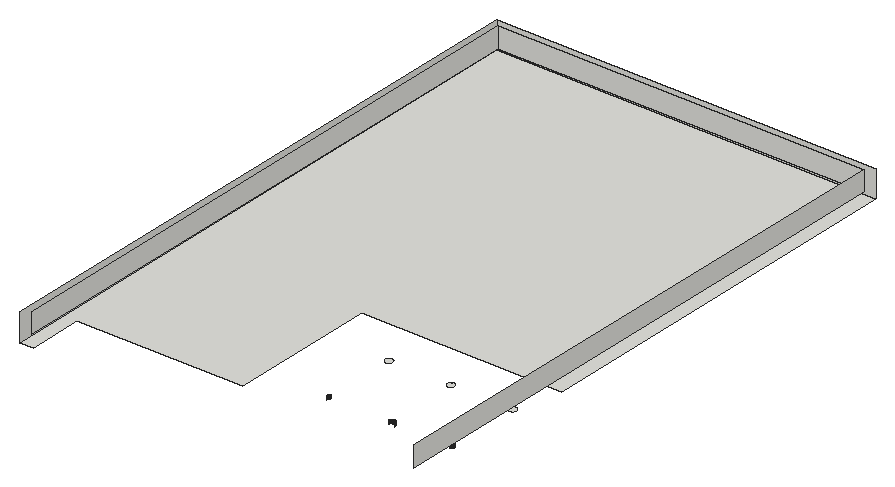
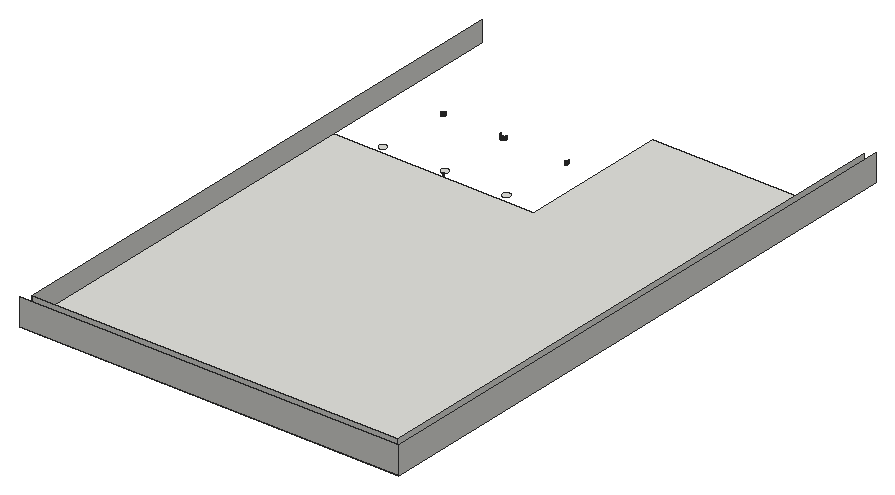
# SketchUp Ruby script. Lengths in inches.
U = 1.inch
M = Sketchup.active_model
def pt(a) = Geom::Point3d.new(a.map { |v| v * U })
def face(e, loops, mat)
  f = e.add_face(loops[0].map { |a| pt(a) })
  loops[1..].each { |l| e.add_face(l.map { |a| pt(a) }).erase! }
  f.material = f.back_material = mat if mat
  f
end
# faces: each face lists its corners as indices into pts; further lists are holes
def faces(e, pts, list, mat = nil) = list.each { |f| face(e, (f[0].is_a?(Array) ? f : [f]).map { |l| l.map { |i| pts[i] } }, mat) }
# xy, xz, yz: faces in a plane at the given z, y or x. An outline is a flat list of corners, or four numbers for a rectangle; further outlines are holes
def ring(l) = l.size == 4 ? [[l[0], l[1]], [l[2], l[1]], [l[2], l[3]], [l[0], l[3]]] : l.each_slice(2).to_a
def flat(e, list, mat, &to3) = list.each { |f| face(e, (f[0].is_a?(Array) ? f : [f]).map { |l| ring(l).map { |u, v| to3.(u, v) } }, mat) }
def xy(e, z, list, mat = nil) = flat(e, list, mat) { |x, y| [x, y, z] }
def xz(e, y, list, mat = nil) = flat(e, list, mat) { |x, z| [x, y, z] }
def yz(e, x, list, mat = nil) = flat(e, list, mat) { |y, z| [x, y, z] }
def lines(e, pts, list) = list.each { |a, b| e.add_line(pt(pts[a]), pt(pts[b])) }
# prism: a flat outline (further loops are holes) pulled along v
def prism(e, loops, v, mat = nil)
  f = face(e, loops, mat); d = Geom::Vector3d.new(v.map { |x| x * U })
  f.pushpull(f.normal.samedirection?(d) ? d.length : -d.length)
end
def box(e, o, s, mat = nil) = prism(e, [[o, [o[0] + s[0], o[1], o[2]], [o[0] + s[0], o[1] + s[1], o[2]], [o[0], o[1] + s[1], o[2]]]], [0, 0, s[2]], mat)
def at(x, y, z, deg = 0) = Geom::Transformation.translation(pt([x, y, z])) * Geom::Transformation.rotation(ORIGIN, Z_AXIS, deg.degrees)
def axes(o, x, y, z) = Geom::Transformation.new([*x, 0, *y, 0, *z, 0, *pt(o).to_a, 1])
def part(name) = M.definitions.add(name)
# library, detail: a bought-in or finely detailed component or shape, given as its bounding box
def library(name, o, s) = part(name).tap { |d| box(d.entities, o, s) }
def detail(e, o, s) = box(e.add_group.entities, o, s)
def put(e, d, t, mat = nil) = e.add_instance(d, t).tap { |i| i.material = mat if mat }
def group(e, t, mat = nil) = e.add_group.tap { |g| g.transformation = t; g.material = mat if mat }.entities
root = M.entities
xy(root,234,[[214.28,317,214.2,317.01,214.12,317.01,213.96,317.03,213.89,317.04,213.73,317.08,213.66,317.09,213.58,317.11,213.5,317.14,213.43,317.16,213.36,317.1875,213.28,317.22,213.14,317.28,213.07,317.3125,213,317.35,212.93,317.39,212.86,317.42,212.79,317.47,212.73,317.51,212.66,317.55,212.36,317.8,212.19,317.97,211.99,318.21,211.95,318.27,211.9,318.34,211.86,318.4,211.74,318.61,211.71,318.68,211.67,318.75,211.61,318.89,211.58,318.97,211.56,319.04,211.53,319.12,211.51,319.19,211.49,319.27,211.47,319.34,211.46,319.42,211.44,319.5,211.43,319.58,211.42,319.65,211.41,319.73,211.41,319.81,211.4,319.89,211.4,320.125,211.41,320.2,211.41,320.28,211.42,320.36,211.43,320.4375,211.44,320.51,211.48,320.67,211.49,320.74,211.51,320.82,211.54,320.9,211.5625,320.97,211.59,321.04,211.62,321.12,211.71,321.33,211.79,321.47,211.82,321.54,211.87,321.61,211.91,321.67,211.95,321.74,212.2,322.04,212.26,322.1,212.3125,322.15,212.37,322.21,212.61,322.41,212.67,322.45,212.74,322.5,212.8,322.54,212.87,322.58,212.9375,322.62,213.01,322.66,213.08,322.69,213.15,322.73,213.29,322.79,213.37,322.82,213.44,322.84,213.52,322.87,213.59,322.89,213.67,322.91,213.74,322.93,213.82,322.94,213.9,322.96,213.98,322.97,214.05,322.98,214.13,322.99,214.21,322.99,214.29,323,214.52,323,214.6,322.99,214.68,322.99,214.84,322.97,214.91,322.96,215.07,322.92,215.14,322.91,215.22,322.89,215.3,322.86,215.37,322.84,215.44,322.8125,215.52,322.78,215.66,322.72,215.73,322.6875,215.8,322.65,215.87,322.61,215.9375,322.58,216.01,322.53,216.07,322.49,216.14,322.45,216.44,322.2,216.61,322.03,216.81,321.79,216.85,321.73,216.9,321.66,216.94,321.6,217.06,321.39,217.09,321.32,217.16,321.18,217.1875,321.11,217.22,321.03,217.24,320.96,217.27,320.88,217.29,320.81,217.31,320.73,217.33,320.66,217.34,320.58,217.36,320.5,217.37,320.42,217.38,320.35,217.39,320.27,217.39,320.19,217.4,320.11,217.4,319.875,217.39,319.8,217.39,319.72,217.38,319.64,217.37,319.5625,217.36,319.49,217.32,319.33,217.31,319.26,217.29,319.18,217.26,319.1,217.24,319.03,217.21,318.96,217.18,318.88,217.09,318.67,217.01,318.53,216.98,318.46,216.93,318.39,216.89,318.33,216.85,318.26,216.6,317.96,216.43,317.79,216.375,317.74,216.25,317.64,216.19,317.59,216.125,317.55,216.0625,317.5,216,317.46,215.79,317.34,215.72,317.31,215.65,317.27,215.51,317.21,215.43,317.18,215.36,317.16,215.28,317.13,215.21,317.11,215.13,317.09,215.06,317.07,214.98,317.06,214.9,317.04,214.82,317.03,214.75,317.02,214.67,317.01,214.59,317.01,214.51,317],[269.08,317,269,317.01,268.92,317.01,268.76,317.03,268.6875,317.04,268.61,317.06,268.53,317.08,268.46,317.09,268.38,317.11,268.3,317.14,268.23,317.16,268.16,317.1875,268.08,317.22,268.01,317.25,267.9375,317.28,267.87,317.3125,267.8,317.35,267.73,317.39,267.66,317.42,267.59,317.47,267.53,317.51,267.46,317.55,267.16,317.8,266.99,317.97,266.79,318.21,266.75,318.27,266.7,318.34,266.66,318.4,266.54,318.61,266.51,318.68,266.47,318.75,266.41,318.89,266.38,318.97,266.36,319.04,266.33,319.12,266.3125,319.19,266.29,319.27,266.27,319.34,266.26,319.42,266.24,319.5,266.23,319.58,266.22,319.65,266.21,319.73,266.21,319.81,266.2,319.89,266.2,320.125,266.21,320.2,266.21,320.28,266.22,320.36,266.23,320.4375,266.24,320.51,266.28,320.67,266.29,320.74,266.3125,320.82,266.34,320.9,266.36,320.97,266.39,321.04,266.42,321.12,266.51,321.33,266.59,321.47,266.625,321.54,266.67,321.61,266.71,321.67,266.75,321.74,267,322.04,267.17,322.21,267.41,322.41,267.47,322.45,267.54,322.5,267.6,322.54,267.81,322.66,267.88,322.69,267.95,322.73,268.09,322.79,268.17,322.82,268.24,322.84,268.32,322.87,268.39,322.89,268.47,322.91,268.54,322.93,268.62,322.94,268.7,322.96,268.78,322.97,268.85,322.98,268.93,322.99,269.01,322.99,269.09,323,269.32,323,269.4,322.99,269.48,322.99,269.64,322.97,269.71,322.96,269.87,322.92,269.94,322.91,270.02,322.89,270.1,322.86,270.17,322.84,270.24,322.8125,270.32,322.78,270.46,322.72,270.53,322.6875,270.6,322.65,270.67,322.61,270.74,322.58,270.81,322.53,270.87,322.49,270.9375,322.45,271.0625,322.35,271.12,322.3,271.24,322.2,271.41,322.03,271.61,321.79,271.65,321.73,271.7,321.66,271.74,321.6,271.86,321.39,271.89,321.32,271.93,321.25,271.99,321.11,272.02,321.03,272.04,320.96,272.07,320.88,272.09,320.81,272.11,320.73,272.13,320.66,272.14,320.58,272.16,320.5,272.17,320.42,272.18,320.35,272.1875,320.27,272.19,320.19,272.2,320.11,272.2,319.875,272.19,319.8,272.1875,319.72,272.18,319.64,272.17,319.5625,272.16,319.49,272.14,319.41,272.125,319.33,272.11,319.26,272.09,319.18,272.0625,319.1,272.04,319.03,272.01,318.96,271.98,318.88,271.89,318.67,271.81,318.53,271.78,318.46,271.73,318.39,271.69,318.33,271.65,318.26,271.4,317.96,271.23,317.79,270.99,317.59,270.93,317.55,270.86,317.5,270.8,317.46,270.59,317.34,270.52,317.31,270.45,317.27,270.31,317.21,270.23,317.18,270.16,317.16,270.08,317.13,270.01,317.11,269.93,317.09,269.86,317.07,269.78,317.06,269.7,317.04,269.55,317.02,269.47,317.01,269.39,317.01,269.3125,317],[323.875,317,323.8,317.01,323.72,317.01,323.64,317.02,323.5625,317.03,323.49,317.04,323.33,317.08,323.26,317.09,323.18,317.11,323.1,317.14,323.03,317.16,322.96,317.1875,322.88,317.22,322.74,317.28,322.67,317.3125,322.6,317.35,322.53,317.39,322.46,317.42,322.39,317.47,322.33,317.51,322.26,317.55,321.96,317.8,321.79,317.97,321.59,318.21,321.55,318.27,321.5,318.34,321.46,318.4,321.34,318.61,321.31,318.68,321.27,318.75,321.21,318.89,321.18,318.97,321.16,319.04,321.13,319.12,321.11,319.19,321.09,319.27,321.07,319.34,321.06,319.42,321.04,319.5,321.03,319.58,321.02,319.65,321.01,319.73,321.01,319.81,321,319.89,321,320.125,321.01,320.2,321.01,320.28,321.02,320.36,321.03,320.4375,321.04,320.51,321.08,320.67,321.09,320.74,321.11,320.82,321.14,320.9,321.16,320.97,321.1875,321.04,321.22,321.12,321.28,321.26,321.3125,321.33,321.35,321.4,321.39,321.47,321.42,321.54,321.47,321.61,321.51,321.67,321.55,321.74,321.8,322.04,321.97,322.21,322.21,322.41,322.27,322.45,322.34,322.5,322.4,322.54,322.61,322.66,322.68,322.69,322.75,322.73,322.89,322.79,322.97,322.82,323.04,322.84,323.12,322.87,323.19,322.89,323.27,322.91,323.34,322.93,323.42,322.94,323.5,322.96,323.58,322.97,323.65,322.98,323.73,322.99,323.81,322.99,323.89,323,324.125,323,324.2,322.99,324.28,322.99,324.36,322.98,324.4375,322.97,324.51,322.96,324.67,322.92,324.74,322.91,324.82,322.89,324.9,322.86,324.97,322.84,325.04,322.8125,325.12,322.78,325.26,322.72,325.33,322.6875,325.4,322.65,325.47,322.61,325.54,322.58,325.61,322.53,325.67,322.49,325.74,322.45,326.04,322.2,326.21,322.03,326.41,321.79,326.45,321.73,326.5,321.66,326.54,321.6,326.66,321.39,326.69,321.32,326.73,321.25,326.79,321.11,326.82,321.03,326.84,320.96,326.87,320.88,326.89,320.81,326.91,320.73,326.93,320.66,326.94,320.58,326.96,320.5,326.97,320.42,326.98,320.35,326.99,320.27,326.99,320.19,327,320.11,327,319.875,326.99,319.8,326.99,319.72,326.98,319.64,326.97,319.5625,326.96,319.49,326.92,319.33,326.91,319.26,326.89,319.18,326.86,319.1,326.84,319.03,326.8125,318.96,326.78,318.88,326.72,318.74,326.6875,318.67,326.65,318.6,326.61,318.53,326.58,318.46,326.53,318.39,326.49,318.33,326.45,318.26,326.2,317.96,326.03,317.79,325.79,317.59,325.73,317.55,325.66,317.5,325.6,317.46,325.39,317.34,325.32,317.31,325.25,317.27,325.11,317.21,325.03,317.18,324.96,317.16,324.88,317.13,324.81,317.11,324.73,317.09,324.66,317.07,324.58,317.06,324.5,317.04,324.42,317.03,324.35,317.02,324.27,317.01,324.19,317.01,324.11,317]])
xy(root,246,[[12,164,12,692,348,692,348,344,171,344,171,212,24,212,24,164]])
xz(root,256.99,[[268.93,231,269.01,234],[269.4,231,269.48,234]])
xz(root,257,[[269.09,231,269.17,234],[269.17,231,269.25,234],[269.25,231,269.32,234]])
xz(root,686,[[18,252,342,270]])
xz(root,692,[[12,246,348,270]])
yz(root,12,[[164,246,692,270]])
yz(root,18,[[170,252,686,270]])
yz(root,342,[[188,252,686,270]])
p = [[211.43,254.4375,231],[211.44,254.51,231],[211.44,254.51,234],[211.43,254.4375,234],[266.22,254.36,231],[266.23,254.4375,231],
  [266.23,254.4375,234],[266.22,254.36,234],[266.24,254.51,231],[266.24,254.51,234],[272.16,254.5,231],[272.17,254.42,231],
  [272.17,254.42,234],[272.16,254.5,234],[321.02,254.36,231],[321.03,254.4375,231],[321.03,254.4375,234],[321.02,254.36,234],
  [321.04,254.51,231],[321.04,254.51,234],[211.46,254.59,231],[211.46,254.59,234],[266.26,254.59,231],[266.26,254.59,234],
  [272.14,254.58,231],[272.14,254.58,234],[321.06,254.59,231],[321.06,254.59,234],[211.48,254.67,231],[211.48,254.67,234],
  [266.28,254.67,231],[266.28,254.67,234],[272.13,254.66,231],[272.13,254.66,234],[321.08,254.67,231],[321.08,254.67,234],
  [211.49,254.74,231],[211.49,254.74,234],[211.51,254.82,231],[211.51,254.82,234],[266.29,254.74,231],[266.29,254.74,234],
  [266.3125,254.82,231],[266.3125,254.82,234],[272.11,254.73,231],[272.11,254.73,234],[272.09,254.81,231],[272.09,254.81,234],
  [321.09,254.74,231],[321.09,254.74,234],[321.11,254.82,231],[321.11,254.82,234],[211.54,254.9,231],[211.54,254.9,234],
  [266.34,254.9,231],[266.34,254.9,234],[272.07,254.88,231],[272.07,254.88,234],[321.14,254.9,231],[321.14,254.9,234],
  [211.5625,254.97,231],[211.5625,254.97,234],[266.36,254.97,231],[266.36,254.97,234],[272.04,254.96,231],[272.04,254.96,234],
  [321.16,254.97,231],[321.16,254.97,234],[211.59,255.04,231],[211.59,255.04,234],[211.62,255.12,231],[211.62,255.12,234],
  [266.39,255.04,231],[266.39,255.04,234],[266.42,255.12,231],[266.42,255.12,234],[272.02,255.03,231],[272.02,255.03,234],
  [271.99,255.11,231],[271.99,255.11,234],[321.1875,255.04,231],[321.1875,255.04,234],[321.22,255.12,231],[321.22,255.12,234],
  [211.65,255.19,231],[211.65,255.19,234],[266.45,255.19,231],[266.45,255.19,234],[271.96,255.18,231],[271.96,255.18,234],
  [321.25,255.19,231],[321.25,255.19,234],[211.68,255.26,231],[211.68,255.26,234],[266.48,255.26,231],[266.48,255.26,234],
  [271.93,255.25,231],[271.93,255.25,234],[321.28,255.26,231],[321.28,255.26,234],[211.71,255.33,231],[211.71,255.33,234],
  [211.75,255.4,231],[211.75,255.4,234],[266.51,255.33,231],[266.51,255.33,234],[266.55,255.4,231],[266.55,255.4,234],
  [271.89,255.32,231],[271.89,255.32,234],[271.86,255.39,231],[271.86,255.39,234],[321.3125,255.33,231],[321.3125,255.33,234],
  [321.35,255.4,231],[321.35,255.4,234],[211.79,255.47,231],[211.79,255.47,234],[266.59,255.47,231],[266.59,255.47,234],
  [271.82,255.46,231],[271.82,255.46,234],[321.39,255.47,231],[321.39,255.47,234],[211.82,255.54,231],[211.82,255.54,234],
  [211.87,255.61,231],[211.87,255.61,234],[266.625,255.54,231],[266.625,255.54,234],[266.67,255.61,231],[266.67,255.61,234],
  [271.74,255.6,231],[271.78,255.53,231],[271.78,255.53,234],[271.74,255.6,234],[321.42,255.54,231],[321.42,255.54,234],
  [321.47,255.61,231],[321.47,255.61,234],[211.91,255.67,231],[211.91,255.67,234],[266.71,255.67,231],[266.71,255.67,234],
  [271.7,255.66,231],[271.7,255.66,234],[321.51,255.67,231],[321.51,255.67,234],[211.95,255.74,231],[211.95,255.74,234],
  [212,255.8,231],[212,255.8,234],[266.75,255.74,231],[266.75,255.74,234],[266.8,255.8,231],[266.8,255.8,234],
  [271.61,255.79,231],[271.65,255.73,231],[271.65,255.73,234],[271.61,255.79,234],[321.55,255.74,231],[321.55,255.74,234],
  [321.6,255.8,231],[321.6,255.8,234],[212.05,255.86,231],[212.05,255.86,234],[266.85,255.86,231],[266.85,255.86,234],
  [271.56,255.85,231],[271.56,255.85,234],[321.65,255.86,231],[321.65,255.86,234],[212.1,255.92,231],[212.1,255.92,234],
  [212.15,255.98,231],[212.15,255.98,234],[266.9,255.92,231],[266.9,255.92,234],[266.95,255.98,231],[266.95,255.98,234],
  [271.51,255.91,231],[271.51,255.91,234],[271.46,255.97,231],[271.46,255.97,234],[321.7,255.92,231],[321.7,255.92,234],
  [321.75,255.98,231],[321.75,255.98,234],[212.2,256.04,231],[212.2,256.04,234],[212.26,256.1,231],[212.26,256.1,234],
  [267,256.04,231],[267,256.04,234],[267.06,256.1,231],[267.06,256.1,234],[271.41,256.03,231],[271.41,256.03,234],
  [271.35,256.09,231],[271.35,256.09,234],[321.8,256.04,231],[321.8,256.04,234],[321.86,256.1,231],[321.86,256.1,234],
  [212.3125,256.15,231],[212.3125,256.15,234],[267.11,256.15,231],[267.11,256.15,234],[271.24,256.2,231],[271.3,256.14,231],
  [271.3,256.14,234],[271.24,256.2,234],[321.91,256.15,231],[321.91,256.15,234],[212.37,256.21,231],[212.37,256.21,234],
  [212.43,256.26,231],[212.43,256.26,234],[267.17,256.21,231],[267.17,256.21,234],[267.23,256.26,231],[267.23,256.26,234],
  [271.18,256.25,231],[271.18,256.25,234],[321.97,256.21,231],[321.97,256.21,234],[322.03,256.26,231],[322.03,256.26,234],
  [212.49,256.31,231],[212.49,256.31,234],[212.55,256.36,231],[212.55,256.36,234],[267.29,256.31,231],[267.29,256.31,234],
  [267.35,256.36,231],[267.35,256.36,234],[271.12,256.3,231],[271.12,256.3,234],[271.0625,256.35,231],[271.0625,256.35,234],
  [322.09,256.31,231],[322.09,256.31,234],[322.15,256.36,231],[322.15,256.36,234],[212.61,256.41,231],[212.61,256.41,234],
  [212.67,256.45,231],[212.67,256.45,234],[267.41,256.41,231],[267.41,256.41,234],[267.47,256.45,231],[267.47,256.45,234],
  [270.9375,256.45,231],[271,256.4,231],[271,256.4,234],[270.9375,256.45,234],[270.87,256.49,231],[270.87,256.49,234],
  [322.21,256.41,231],[322.21,256.41,234],[322.27,256.45,231],[322.27,256.45,234],[212.74,256.5,231],[212.74,256.5,234],
  [212.8,256.54,231],[212.8,256.54,234],[212.87,256.58,231],[212.87,256.58,234],[267.54,256.5,231],[267.54,256.5,234],
  [267.6,256.54,231],[267.6,256.54,234],[267.67,256.58,231],[267.67,256.58,234],[270.74,256.58,231],[270.81,256.53,231],
  [270.81,256.53,234],[270.74,256.58,234],[322.34,256.5,231],[322.34,256.5,234],[322.4,256.54,231],[322.4,256.54,234],
  [322.47,256.58,231],[322.47,256.58,234],[212.9375,256.62,231],[212.9375,256.62,234],[213.01,256.66,231],[213.01,256.66,234],
  [267.74,256.62,231],[267.74,256.62,234],[267.81,256.66,231],[267.81,256.66,234],[270.6,256.65,231],[270.67,256.61,231],
  [270.67,256.61,234],[270.6,256.65,234],[322.54,256.62,231],[322.54,256.62,234],[322.61,256.66,231],[322.61,256.66,234],
  [213.08,256.69,231],[213.08,256.69,234],[213.15,256.73,231],[213.15,256.73,234],[213.22,256.76,231],[213.22,256.76,234],
  [267.88,256.69,231],[267.88,256.69,234],[267.95,256.73,231],[267.95,256.73,234],[268.02,256.76,231],[268.02,256.76,234],
  [270.39,256.75,231],[270.46,256.72,231],[270.46,256.72,234],[270.39,256.75,234],[270.53,256.6875,231],[270.53,256.6875,234],
  [322.68,256.69,231],[322.68,256.69,234],[322.75,256.73,231],[322.75,256.73,234],[322.82,256.76,231],[322.82,256.76,234],
  [213.29,256.79,231],[213.29,256.79,234],[213.37,256.82,231],[213.37,256.82,234],[213.44,256.84,231],[213.44,256.84,234],
  [213.52,256.87,231],[213.52,256.87,234],[268.09,256.79,231],[268.09,256.79,234],[268.17,256.82,231],[268.17,256.82,234],
  [268.24,256.84,231],[268.24,256.84,234],[268.32,256.87,231],[268.32,256.87,234],[270.1,256.86,231],[270.17,256.84,231],
  [270.17,256.84,234],[270.1,256.86,234],[270.24,256.8125,231],[270.32,256.78,231],[270.32,256.78,234],[270.24,256.8125,234],
  [322.89,256.79,231],[322.89,256.79,234],[322.97,256.82,231],[322.97,256.82,234],[323.04,256.84,231],[323.04,256.84,234],
  [323.12,256.87,231],[323.12,256.87,234],[268.39,256.89,231],[268.39,256.89,234],[268.47,256.91,231],[268.47,256.91,234],
  [268.54,256.93,231],[268.54,256.93,234],[268.62,256.94,231],[268.62,256.94,234],[268.7,256.96,231],[268.7,256.96,234],
  [269.71,256.96,231],[269.79,256.94,231],[269.79,256.94,234],[269.71,256.96,234],[269.87,256.92,231],[269.87,256.92,234],
  [269.94,256.91,231],[270.02,256.89,231],[270.02,256.89,234],[269.94,256.91,234],[268.78,256.97,231],[268.78,256.97,234],
  [268.85,256.98,231],[268.85,256.98,234],[268.93,256.99,231],[268.93,256.99,234],[269.01,256.99,231],[269.09,257,231],
  [269.09,257,234],[269.01,256.99,234],[269.32,257,231],[269.4,256.99,231],[269.4,256.99,234],[269.32,257,234],
  [269.48,256.99,231],[269.56,256.98,231],[269.56,256.98,234],[269.48,256.99,234],[269.64,256.97,231],[269.64,256.97,234],
  [267.67,322.58,231],[267.74,322.62,231],[267.74,322.62,234],[267.67,322.58,234],[267.81,322.66,231],[267.81,322.66,234],
  [267.88,322.69,231],[267.88,322.69,234],[267.95,322.73,231],[267.95,322.73,234],[268.02,322.76,231],[268.02,322.76,234],
  [268.09,322.79,231],[268.09,322.79,234],[268.17,322.82,231],[268.17,322.82,234],[268.24,322.84,231],[268.24,322.84,234],
  [268.32,322.87,231],[268.32,322.87,234]]
faces(root,p,[[0,1,2,3],[4,5,6,7],[5,8,9,6],[10,11,12,13],[14,15,16,17],[15,18,19,16],[1,20,21,2],[8,22,23,9],
  [24,10,13,25],[18,26,27,19],[20,28,29,21],[22,30,31,23],[32,24,25,33],[26,34,35,27],[28,36,37,29],[36,38,39,37],
  [30,40,41,31],[40,42,43,41],[44,32,33,45],[46,44,45,47],[34,48,49,35],[48,50,51,49],[38,52,53,39],[42,54,55,43],
  [56,46,47,57],[50,58,59,51],[52,60,61,53],[54,62,63,55],[64,56,57,65],[58,66,67,59],[60,68,69,61],[68,70,71,69],
  [62,72,73,63],[72,74,75,73],[76,64,65,77],[78,76,77,79],[66,80,81,67],[80,82,83,81],[70,84,85,71],[74,86,87,75],
  [88,78,79,89],[82,90,91,83],[84,92,93,85],[86,94,95,87],[96,88,89,97],[90,98,99,91],[92,100,101,93],[100,102,103,101],
  [94,104,105,95],[104,106,107,105],[108,96,97,109],[110,108,109,111],[98,112,113,99],[112,114,115,113],[102,116,117,103],[106,118,119,107],
  [120,110,111,121],[114,122,123,115],[116,124,125,117],[124,126,127,125],[118,128,129,119],[128,130,131,129],[132,133,134,135],[133,120,121,134],
  [122,136,137,123],[136,138,139,137],[126,140,141,127],[130,142,143,131],[144,132,135,145],[138,146,147,139],[140,148,149,141],[148,150,151,149],
  [142,152,153,143],[152,154,155,153],[156,157,158,159],[157,144,145,158],[146,160,161,147],[160,162,163,161],[150,164,165,151],[154,166,167,155],
  [168,156,159,169],[162,170,171,163],[164,172,173,165],[172,174,175,173],[166,176,177,167],[176,178,179,177],[180,168,169,181],[182,180,181,183],
  [170,184,185,171],[184,186,187,185],[174,188,189,175],[188,190,191,189],[178,192,193,179],[192,194,195,193],[196,182,183,197],[198,196,197,199],
  [186,200,201,187],[200,202,203,201],[190,204,205,191],[194,206,207,195],[208,209,210,211],[209,198,199,210],[202,212,213,203],[204,214,215,205],
  [214,216,217,215],[206,218,219,207],[218,220,221,219],[222,208,211,223],[212,224,225,213],[224,226,227,225],[216,228,229,217],[228,230,231,229],
  [220,232,233,221],[232,234,235,233],[236,222,223,237],[238,236,237,239],[226,240,241,227],[240,242,243,241],[230,244,245,231],[244,246,247,245],
  [234,248,249,235],[248,250,251,249],[252,253,254,255],[256,252,255,257],[253,238,239,254],[242,258,259,243],[258,260,261,259],[246,262,263,247],
  [262,264,265,263],[264,266,267,265],[250,268,269,251],[268,270,271,269],[270,272,273,271],[274,275,276,277],[275,256,257,276],[260,278,279,261],
  [278,280,281,279],[280,282,283,281],[266,284,285,267],[284,286,287,285],[272,288,289,273],[288,290,291,289],[292,293,294,295],[293,274,277,294],
  [282,296,297,283],[296,298,299,297],[286,300,301,287],[300,302,303,301],[302,304,305,303],[290,306,307,291],[306,308,309,307],[308,310,311,309],
  [312,313,314,315],[316,292,295,317],[313,316,317,314],[298,318,319,299],[318,320,321,319],[320,322,323,321],[304,324,325,305],[324,326,327,325],
  [326,328,329,327],[328,330,331,329],[310,332,333,311],[332,334,335,333],[334,336,337,335],[336,338,339,337],[340,341,342,343],[344,345,346,347],
  [341,344,347,342],[345,312,315,346],[322,348,349,323],[348,350,351,349],[350,352,353,351],[352,354,355,353],[338,356,357,339],[356,358,359,357],
  [358,360,361,359],[360,362,363,361],[362,364,365,363],[366,367,368,369],[367,370,371,368],[372,373,374,375],[370,372,375,371],[373,340,343,374],
  [364,376,377,365],[376,378,379,377],[378,380,381,379],[382,383,384,385],[386,387,388,389],[390,391,392,393],[394,366,369,395],[391,394,395,392],
  [396,397,398,399],[397,400,401,398],[400,402,403,401],[402,404,405,403],[404,406,407,405],[406,408,409,407],[408,410,411,409],[410,412,413,411],
  [412,414,415,413]])
